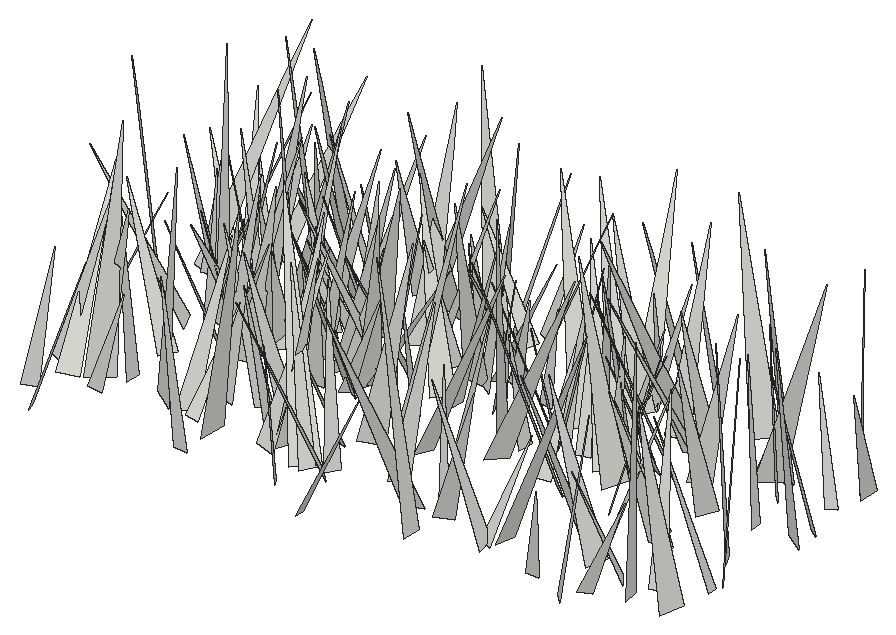
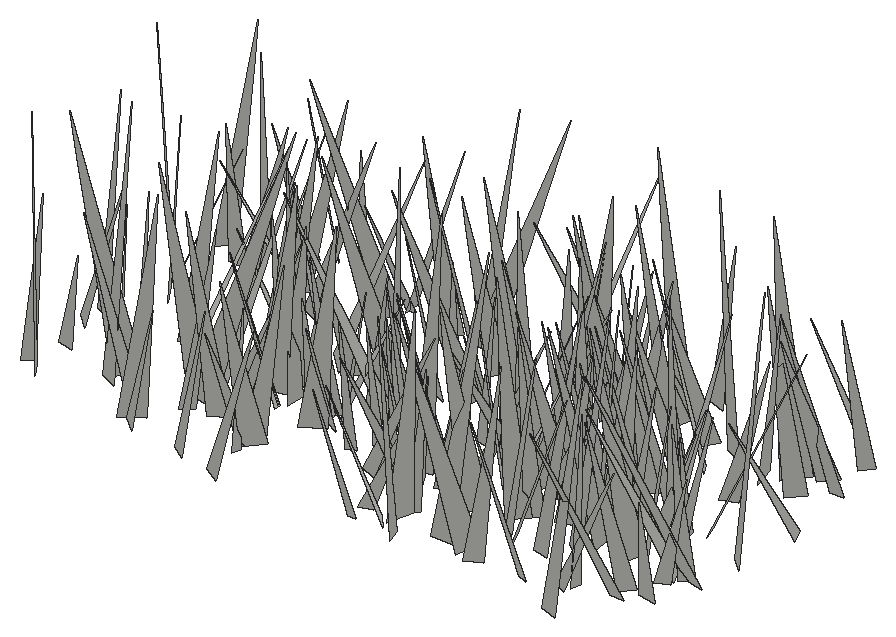
# SketchUp Ruby script. Lengths in inches.
U = 1.inch
M = Sketchup.active_model
def pt(a) = Geom::Point3d.new(a.map { |v| v * U })
def face(e, loops, mat)
  f = e.add_face(loops[0].map { |a| pt(a) })
  loops[1..].each { |l| e.add_face(l.map { |a| pt(a) }).erase! }
  f.material = f.back_material = mat if mat
  f
end
# faces: each face lists its corners as indices into pts; further lists are holes
def faces(e, pts, list, mat = nil) = list.each { |f| face(e, (f[0].is_a?(Array) ? f : [f]).map { |l| l.map { |i| pts[i] } }, mat) }
# xy, xz, yz: faces in a plane at the given z, y or x. An outline is a flat list of corners, or four numbers for a rectangle; further outlines are holes
def ring(l) = l.size == 4 ? [[l[0], l[1]], [l[2], l[1]], [l[2], l[3]], [l[0], l[3]]] : l.each_slice(2).to_a
def flat(e, list, mat, &to3) = list.each { |f| face(e, (f[0].is_a?(Array) ? f : [f]).map { |l| ring(l).map { |u, v| to3.(u, v) } }, mat) }
def xy(e, z, list, mat = nil) = flat(e, list, mat) { |x, y| [x, y, z] }
def xz(e, y, list, mat = nil) = flat(e, list, mat) { |x, z| [x, y, z] }
def yz(e, x, list, mat = nil) = flat(e, list, mat) { |y, z| [x, y, z] }
def lines(e, pts, list) = list.each { |a, b| e.add_line(pt(pts[a]), pt(pts[b])) }
# prism: a flat outline (further loops are holes) pulled along v
def prism(e, loops, v, mat = nil)
  f = face(e, loops, mat); d = Geom::Vector3d.new(v.map { |x| x * U })
  f.pushpull(f.normal.samedirection?(d) ? d.length : -d.length)
end
def box(e, o, s, mat = nil) = prism(e, [[o, [o[0] + s[0], o[1], o[2]], [o[0] + s[0], o[1] + s[1], o[2]], [o[0], o[1] + s[1], o[2]]]], [0, 0, s[2]], mat)
def at(x, y, z, deg = 0) = Geom::Transformation.translation(pt([x, y, z])) * Geom::Transformation.rotation(ORIGIN, Z_AXIS, deg.degrees)
def axes(o, x, y, z) = Geom::Transformation.new([*x, 0, *y, 0, *z, 0, *pt(o).to_a, 1])
def part(name) = M.definitions.add(name)
# library, detail: a bought-in or finely detailed component or shape, given as its bounding box
def library(name, o, s) = part(name).tap { |d| box(d.entities, o, s) }
def detail(e, o, s) = box(e.add_group.entities, o, s)
def put(e, d, t, mat = nil) = e.add_instance(d, t).tap { |i| i.material = mat if mat }
def group(e, t, mat = nil) = e.add_group.tap { |g| g.transformation = t; g.material = mat if mat }.entities
root = M.entities
c1 = part("fur_instance\#9")
p = [[0.8125,0,1.79],[0.67,-0.02,1.48],[0,-0.11,0],[0,0.11,0]]
faces(c1.entities,p,[[0,1,2,3]])
put(root,c1,axes([525.23,306.68,-21.66],[4.11341,0.99659,0.14821],[0.94897,-4.04143,0.83763],[-0.33855,0.78037,4.1487]))
put(root,c1,axes([506.24,306.79,-21.66],[4.19181,1.99584,0.5753],[1.88629,-4.2003,0.82769],[-0.86965,0.50967,4.56832]))
put(root,c1,axes([515.68,308.2,-21.66],[-1.40726,-4.75955,2.034],[-5.17479,1.24906,-0.65748],[-0.10975,2.13481,4.91949]))
put(root,c1,axes([539.56,309.3,-21.66],[0.99148,-3.49866,0.36174],[-3.47594,-0.91715,0.65665],[0.53788,0.52224,3.57665]))
put(root,c1,axes([523.57,310.96,-21.66],[-4.47092,-4.93614,0.16266],[-4.90041,4.46105,0.68268],[0.61475,-0.33851,6.62484]))
put(root,c1,axes([504.69,308.63,-21.66],[-2.17172,3.54056,2.13295],[3.72846,2.71807,-0.7156],[1.78427,-1.37037,4.09143]))
put(root,c1,axes([529.65,311.23,-21.66],[0.11863,-7.1905,0.64579],[-7.08435,-0.24031,-1.37429],[-1.39009,0.61104,7.05894]))
put(root,c1,axes([522,308.61,-21.66],[-3.20539,-1.99252,1.2784],[-2.28309,3.17085,-0.78241],[0.62603,1.36182,3.69222]))
put(root,c1,axes([543.06,309.57,-21.66],[3.00481,-2.76961,0.12717],[-2.71494,-2.90128,0.96303],[0.56213,0.79222,3.97142]))
put(root,c1,axes([542.36,308.125,-21.66],[3.86177,3.77021,1.4507],[3.73701,-4.09632,0.69796],[-1.5342,-0.48777,5.35169]))
put(root,c1,axes([535.49,310.27,-21.66],[-5.30182,-0.75056,0.88287],[-0.65483,5.35184,0.61739],[0.95603,-0.49663,5.31898]))
put(root,c1,axes([531.5,308.73,-21.66],[-7.85501,-1.13743,1.66782],[-1.3997,7.89692,-1.20666],[1.45472,1.45652,7.84468]))
put(root,c1,axes([548.03,311,-21.66],[-6.01027,1.97565,2.91231],[2.62602,6.35479,1.10849],[2.3428,-2.05464,6.22879]))
put(root,c1,axes([515.82,310.82,-21.66],[7.89082,-0.9052,1.78608],[-0.78265,-8.07818,-0.63641],[-1.84308,-0.44515,7.91703]))
put(root,c1,axes([531.8,311.22,-21.66],[3.60736,-4.41491,0.21347],[-4.38405,-3.53869,0.89879],[0.56311,0.73233,5.62998]))
put(root,c1,axes([507.74,310.5625,-21.66],[1.20072,-3.47995,0.99765],[-3.52529,-0.88496,1.15597],[0.82322,1.28603,3.49507]))
put(root,c1,axes([543.75,312.04,-21.66],[-3.41692,-2.65793,0.41527],[-2.50813,3.39027,1.06197],[0.9728,-0.5949,4.19669]))
put(root,c1,axes([535.33,310.45,-21.66],[0.85166,3.52496,0.51911],[3.494,-0.72175,-0.83136],[0.69768,-0.68839,3.5298]))
put(root,c1,axes([511.42,312.01,-21.66],[-3.32783,-6.52848,3.29816],[-6.89122,4.01297,0.99019],[2.45153,2.41834,7.26051]))
put(root,c1,axes([541.49,312.54,-21.66],[-5.54142,2.04017,2.02802],[2.50487,5.58649,1.22443],[1.41448,-1.90035,5.77671]))
put(root,c1,axes([545.33,310.76,-21.66],[-6.71268,-1.89599,2.76742],[-2.51748,6.93875,-1.3526],[2.21714,2.13833,6.8429]))
put(root,c1,axes([507.07,311.85,-21.66],[-5.12716,5.45276,3.67809],[5.84452,5.9162,-0.62364],[3.01704,-2.19425,7.45865]))
put(root,c1,axes([535.95,311.42,-21.66],[7.40622,-0.19557,0.80001],[-0.28757,-7.3972,0.85392],[-0.77173,0.87956,7.35943]))
put(root,c1,axes([522.49,310.92,-21.66],[-5.52094,1.92393,0.48296],[1.85996,5.5174,-0.71721],[0.68943,0.52184,5.80241]))
put(root,c1,axes([519.83,312.03,-21.66],[5.84499,-0.86217,1.83487],[-1.09003,-6.05756,0.62599],[-1.70936,0.91471,5.87498]))
put(root,c1,axes([505.89,313.43,-21.66],[3.45559,-4.90486,0.92565],[-4.98413,-3.32981,0.96246],[0.2699,1.30779,5.9222]))
put(root,c1,axes([513.93,311.37,-21.66],[-0.30009,3.62925,0.24074],[3.53668,0.34756,-0.831],[0.84929,-0.16496,3.54556]))
put(root,c1,axes([523.67,311.5625,-21.66],[-5.20641,1.3754,0.94823],[1.21962,5.25029,-0.91901],[1.14166,0.66356,5.30602]))
put(root,c1,axes([522.17,311.0625,-21.66],[-4.81407,6.51041,0.79127],[6.55623,4.75265,0.78417],[-0.16528,-1.10168,8.05889]))
put(root,c1,axes([504.21,311.87,-21.66],[1.48764,5.46016,1.29529],[5.56167,-1.25605,-1.09283],[0.74757,-1.52092,5.55267]))
put(root,c1,axes([519.22,311.18,-21.66],[1.31333,6.20143,0.89],[6.24264,-1.21867,-0.72041],[0.52849,-1.01577,6.2979]))
put(root,c1,axes([539.47,314.21,-21.66],[-1.836,-5.36618,0.72675],[-5.38286,1.72484,-0.86298],[-0.59066,0.96126,5.60554]))
put(root,c1,axes([513.17,311.84,-21.66],[-3.03856,4.16793,1.35783],[3.96538,3.31773,-1.3102],[1.86846,-0.26309,4.98878]))
put(root,c1,axes([517.71,313.45,-21.66],[-1.21907,-3.82959,1.50139],[-4.09681,0.98993,-0.80143],[-0.36895,1.66143,3.93822]))
put(root,c1,axes([505.54,310.92,-21.66],[-3.21539,5.33291,0.27404],[5.21793,3.20577,-1.16191],[1.13501,0.36996,6.11789]))
put(root,c1,axes([530.96,312.28,-21.66],[-3.9297,0.38452,0.60241],[0.18265,3.7953,-1.23109],[0.69093,1.18368,3.75164]))
put(root,c1,axes([527.22,312.97,-21.66],[4.47757,-3.00826,2.16701],[-3.51648,-4.52249,0.98776],[-1.1747,2.07164,5.30307]))
put(root,c1,axes([508.57,312.87,-21.66],[-5.92753,-0.80933,1.51712],[-1.07571,5.99367,-1.00549],[1.34146,1.2301,5.89742]))
put(root,c1,axes([522.33,314.2,-21.66],[-2.45002,-3.17903,0.27674],[-3.09062,2.27713,-1.20338],[-0.79426,0.94543,3.82893]))
put(root,c1,axes([546.05,312.3,-21.66],[-0.40963,5.6712,0.85204],[5.69515,0.30195,0.72827],[-0.67361,-0.89587,5.63914]))
put(root,c1,axes([519.03,313.05,-21.66],[-3.21117,5.73542,2.2751],[5.803,3.67883,-1.08356],[2.09673,-1.39782,6.48325]))
put(root,c1,axes([517.64,315.1875,-21.66],[-5.01187,1.13995,1.85475],[1.60842,5.07616,1.22637],[1.46717,-1.67079,4.99142]))
put(root,c1,axes([511.62,314.23,-21.66],[5.2265,3.38981,1.10604],[3.55749,-5.09026,-1.20993],[-0.2416,-1.62138,6.11091]))
put(root,c1,axes([513.7,314.26,-21.66],[1.63751,6.97927,2.94123],[7.53115,-1.18196,-1.38823],[0.80173,-3.15202,7.03309]))
put(root,c1,axes([548.45,314.0625,-21.66],[-4.94313,-1.68267,0.02369],[-1.64372,4.81198,-1.18726],[-0.36076,1.13137,5.08492]))
put(root,c1,axes([516.32,314.75,-21.66],[0.21554,-5.31829,2.18174],[-5.56977,-0.73327,-1.23719],[-1.42193,2.0661,5.17688]))
put(root,c1,axes([542.6875,316.59,-21.66],[1.51534,-5.37644,0.92666],[-5.31705,-1.67082,-0.99923],[-1.22223,0.60275,5.49581]))
put(root,c1,axes([548.05,315.53,-21.66],[-5.21121,-4.35385,3.58957],[-4.50193,6.15376,0.92827],[3.40202,1.4741,6.72689]))
put(root,c1,axes([541.59,312.71,-21.66],[4.07971,3.91858,0.07723],[3.79656,-3.97882,1.32677],[-0.97331,0.90496,5.499]))
put(root,c1,axes([523.4,315.33,-21.66],[4.4224,-5.22883,1.99199],[-5.58659,-4.26873,1.19762],[-0.31423,2.30295,6.7427]))
put(root,c1,axes([512.45,315.42,-21.66],[4.92372,-1.23429,0.65682],[-1.32256,-4.89156,0.72207],[-0.45359,0.86432,5.02445]))
put(root,c1,axes([536.63,317.3,-21.66],[3.04717,-2.22298,0.43436],[-2.028,-3.00193,-1.13631],[-1.00873,-0.67996,3.59662]))
put(root,c1,axes([542.6,317.14,-21.66],[-4.67386,-0.0885,1.27111],[0.2568,4.66814,1.26925],[1.24804,-1.29194,4.49909]))
put(root,c1,axes([510.14,318.6,-21.66],[-2.61623,-5.06997,0.16776],[-4.93297,2.58676,1.24576],[1.18261,-0.42604,5.56752]))
put(root,c1,axes([508.39,316.18,-21.66],[-3.73959,3.61146,1.09906],[3.77498,3.58144,1.07604],[0.00944,-1.53809,5.08619]))
put(root,c1,axes([543.7,316.25,-21.66],[-3.57996,-1.2077,0.30439],[-1.24532,3.48547,-0.8173],[0.0195,0.87192,3.68872]))
put(root,c1,axes([534.96,317.53,-21.66],[-5.01465,-5.39389,0.78065],[-5.43536,4.87162,-1.25473],[-0.40033,1.42249,7.25716]))
put(root,c1,axes([518.89,319.13,-21.66],[-2.89154,-5.8907,0.51675],[-5.81601,2.937,0.93617],[1.06836,0.04534,6.49499]))
put(root,c1,axes([526.29,316.31,-21.66],[6.61677,-1.08212,0.53072],[-1.15649,-6.53431,1.0953],[-0.3394,1.16883,6.6146]))
put(root,c1,axes([516.71,318.57,-21.66],[1.30695,-5.86281,0.96642],[-5.89292,-1.15208,0.98022],[0.76158,1.14664,5.9262]))
put(root,c1,axes([528.02,317.09,-21.66],[2.95558,3.83246,1.3061],[4.0436,-2.87668,-0.7093],[-0.20723,-1.47175,4.78749]))
put(root,c1,axes([512.33,318.21,-21.66],[4.00541,-4.88826,1.49079],[-5.10449,-3.91872,0.86522],[-0.24835,1.7057,6.26017]))
put(root,c1,axes([546.9,317.29,-21.66],[-5.34444,-2.84039,2.21318],[-3.30562,5.4408,-0.99979],[1.42788,1.96442,5.96919]))
put(root,c1,axes([506.96,319.625,-21.66],[-5.82237,-2.50943,0.01956],[-2.48564,5.77362,0.82736],[0.34528,-0.75212,6.28591]))
put(root,c1,axes([529.86,318.33,-21.66],[6.60673,-3.01857,0.44503],[-3.04917,-6.49303,1.22551],[0.11127,1.29906,7.15953]))
put(root,c1,axes([503.01,316.87,-21.66],[4.04294,1.47662,0.10602],[1.40514,-3.92456,1.07725],[-0.46609,0.97696,4.16717]))
put(root,c1,axes([512.49,319.57,-21.66],[1.67883,-4.20753,0.33675],[-4.18563,-1.61266,0.71764],[0.54516,0.57551,4.47289]))
put(root,c1,axes([519.27,320.28,-21.66],[6.44633,-3.37101,0.63256],[-3.2949,-6.46051,-0.8512],[-0.95262,-0.46602,7.22457]))
put(root,c1,axes([523.14,319.53,-21.66],[-1.38247,-3.90181,0.99129],[-3.91317,1.54858,0.63797],[0.94545,0.70412,4.09003]))
put(root,c1,axes([512.81,320.72,-21.66],[4.57924,-4.33247,0.58798],[-4.22206,-4.60304,-1.03525],[-1.13589,-0.35667,6.21836]))
put(root,c1,axes([518.7,318.98,-21.66],[3.23817,-2.36152,0.30304],[-2.37388,-3.16317,0.7165],[0.18248,0.75624,3.94324]))
put(root,c1,axes([515.875,319.8,-21.66],[3.30583,-2.31707,0.74955],[-2.21165,-3.38553,-0.71128],[-1.01942,-0.16893,3.97384]))
put(root,c1,axes([524.41,317.23,-21.66],[1.50713,3.43781,0.3216],[3.3001,-1.53741,0.96906],[-1.01552,0.10596,3.62641]))
put(root,c1,axes([523.75,317.8,-21.66],[-3.45696,-5.56122,4.74392],[-6.59951,4.63089,0.61955],[3.14299,3.60698,6.51874]))
put(root,c1,axes([542.74,320.71,-21.66],[4.44508,-4.04211,0.97735],[-3.87336,-4.54492,-1.18043],[-1.51359,-0.24009,5.89101]))
put(root,c1,axes([538.5,317.4,-21.66],[3.62249,2.81644,0.55831],[2.6251,-3.61284,1.19278],[-1.16313,0.61769,4.43081]))
put(root,c1,axes([533.35,318.03,-21.66],[-1.89071,3.52857,0.74513],[3.44423,2.01617,-0.80816],[1.06925,-0.25501,3.92077]))
put(root,c1,axes([536.8,320.03,-21.66],[-6.28621,2.90163,2.83322],[3.4688,6.55463,0.9835],[2.10096,-2.14018,6.85337]))
put(root,c1,axes([519.8125,321.31,-21.66],[-5.72076,-3.26575,0.35826],[-3.1922,5.6955,0.94426],[0.77675,-0.64548,6.51924]))
put(root,c1,axes([514.8,319.24,-21.66],[2.68991,-2.47286,1.2383],[-2.72716,-2.65872,0.6147],[-0.45937,1.30393,3.60178]))
put(root,c1,axes([528.72,320.23,-21.66],[6.72646,1.81373,2.96578],[2.30607,-7.16166,-0.85049],[-2.60144,-1.65881,6.91459]))
put(root,c1,axes([530.28,320.27,-21.66],[3.55115,-1.15094,1.45453],[-0.93925,-3.82501,-0.73353],[-1.59941,-0.30919,3.66022]))
put(root,c1,axes([520.47,320.61,-21.66],[1.50872,-3.69838,0.31644],[-3.67115,-1.43625,0.71715],[0.54852,0.55997,3.92937]))
put(root,c1,axes([510.64,318.49,-21.66],[5.6278,2.51424,1.57514],[2.22036,-5.80941,1.3399],[-1.96786,0.63554,6.01649]))
put(root,c1,axes([517.78,320.11,-21.66],[-0.77592,-4.15559,2.31409],[-4.39268,1.52537,1.26634],[1.82437,1.90534,4.03328]))
put(root,c1,axes([503.63,321.42,-21.66],[-5.15951,-5.90719,2.53837],[-5.9684,5.61072,0.92562],[2.3909,1.25844,7.78837]))
put(root,c1,axes([538.63,322.8125,-21.66],[-4.50054,-5.78959,0.45114],[-5.68851,4.51005,1.13049],[1.1678,-0.3432,7.24542]))
put(root,c1,axes([548.48,321.16,-21.66],[-3.10043,-5.65859,2.0595],[-5.81568,3.41455,0.62657],[1.56175,1.48157,6.42182]))
put(root,c1,axes([508.82,321.92,-21.66],[1.51991,-3.61395,0.26794],[-3.4425,-1.53065,-1.11749],[-1.13207,-0.1975,3.75792]))
put(root,c1,axes([509.875,320.1,-21.66],[-3.12705,-1.8127,0.50032],[-1.87769,2.95706,-1.02213],[-0.10232,1.13341,3.46693]))
put(root,c1,axes([521.29,321.94,-21.66],[-1.6318,-4.41068,0.10105],[-4.3461,1.58854,-0.8456],[-0.75876,0.38671,4.62621]))
put(root,c1,axes([535.83,321.03,-21.66],[0.28341,4.29415,2.46111],[4.89058,0.13603,-0.80051],[0.76092,-2.47364,4.22839]))
put(root,c1,axes([537.6875,320.58,-21.66],[-3.61019,-4.99925,2.09321],[-5.40705,3.49453,-0.97958],[0.37125,2.28107,6.08822]))
put(root,c1,axes([540.94,323.39,-21.66],[-5.31992,-4.92486,0.01845],[-4.88394,5.27914,0.91325],[0.63384,-0.65774,7.19179]))
put(root,c1,axes([512.74,320.28,-21.66],[-2.01026,5.06538,1.49078],[5.275,1.85579,0.80751],[-0.23431,-1.67916,5.38954]))
put(root,c1,axes([518.76,321.62,-21.66],[-2.91318,-3.12111,0.33199],[-3.12229,2.8354,-0.74159],[-0.32068,0.74655,4.20452]))
put(root,c1,axes([517.14,320.71,-21.66],[6.46627,-2.11143,1.67342],[-2.36842,-6.52888,0.91405],[-1.28416,1.40953,6.74057]))
put(root,c1,axes([515.45,320.88,-21.66],[5.24089,-0.83273,1.62957],[-1.05437,-5.41429,0.62423],[-1.49573,0.89885,5.2698]))
put(root,c1,axes([534.05,322.27,-21.66],[6.7511,0.38921,2.10678],[0.68602,-6.99103,-0.90679],[-2.02963,-1.06837,6.70124]))
put(root,c1,axes([519.35,320.49,-21.66],[4.38555,-0.36882,0.03632],[-0.36139,-4.16033,1.38975],[0.08213,1.3878,4.17584]))
put(root,c1,axes([531.47,321.92,-21.66],[5.91305,2.63208,1.30513],[2.84881,-5.85376,-1.10147],[-0.71801,-1.54954,6.37799]))
put(root,c1,axes([508.86,320.41,-21.66],[2.99088,7.34321,2.70362],[7.47912,-3.53374,1.32409],[-2.30112,-1.94104,7.81761]))
put(root,c1,axes([530.29,322.79,-21.66],[-2.2334,-3.12116,0.78897],[-3.02774,2.36275,0.77617],[1.09405,0.16724,3.75863]))
put(root,c1,axes([531.11,321.87,-21.66],[-3.78552,-3.06993,0.30173],[-3.01727,3.58565,-1.37288],[-0.64154,1.25071,4.67652]))
put(root,c1,axes([545.77,321.22,-21.66],[-4.75488,-0.89522,1.48594],[-1.16705,4.85843,-0.80746],[1.28353,1.10117,4.77057]))
put(root,c1,axes([537.71,322.61,-21.66],[-2.11494,-3.26023,0.3236],[-3.25153,2.04149,-0.68318],[-0.40176,0.64034,3.82562]))
put(root,c1,axes([507.64,320.73,-21.66],[-4.10668,0.43412,1.0008],[0.12519,4.05996,-1.24738],[1.0837,1.17608,3.93666]))
put(root,c1,axes([509.49,321.6,-21.66],[3.29943,5.39851,1.49465],[5.593,-3.07886,-1.22601],[0.31023,-1.9081,6.20701]))
put(root,c1,axes([523.73,324.16,-21.66],[0.64901,-7.30772,0.94418],[-7.33385,-0.54888,0.79295],[0.71332,1.00569,7.2935]))
put(root,c1,axes([531.41,322.14,-21.66],[-0.36242,4.3186,2.109],[4.6668,0.82166,-0.88056],[1.14855,-1.97588,4.24338]))
put(root,c1,axes([514.19,323.77,-21.66],[-2.66612,-3.28273,0.28859],[-3.19335,2.6653,0.81637],[0.81369,-0.29607,4.14946]))
put(root,c1,axes([514.14,320.26,-21.66],[2.11808,6.39246,0.96016],[6.39192,-2.22182,0.69185],[-0.96378,-0.68681,6.6986]))
put(root,c1,axes([519.23,322.48,-21.66],[4.62058,2.87983,1.50344],[3.15499,-4.60106,-0.88304],[-0.77446,-1.56215,5.37246]))
put(root,c1,axes([535.46,320.94,-21.66],[-3.34888,5.66427,0.75226],[5.70524,3.26636,0.80369],[-0.31635,-1.05439,6.53093]))
put(root,c1,axes([548.75,322.59,-21.66],[-3.27995,-3.84872,1.10692],[-4.00472,3.15616,-0.89264],[0.01123,1.42196,4.97734]))
put(root,c1,axes([513.25,321.55,-21.66],[-6.49961,-2.89491,2.26898],[-3.37847,6.5202,-1.35892],[1.4542,2.20912,6.98418]))
put(root,c1,axes([528.58,320.72,-21.66],[7.17048,3.0592,0.30714],[3.02615,-7.16002,0.66735],[-0.54355,0.49421,7.76718]))
put(root,c1,axes([513.13,322.95,-21.66],[3.69206,0.52175,1.19179],[0.74035,-3.79133,-0.63373],[-1.0698,-0.8231,3.6745]))
put(root,c1,axes([526.38,323.17,-21.66],[-1.07299,-3.39329,1.1863],[-3.30809,1.41653,1.05972],[1.4065,0.74301,3.39746]))
put(root,c1,axes([518.68,322.47,-21.66],[-4.50374,-2.5863,0.2222],[-2.55985,4.35118,-1.23954],[-0.43072,1.18335,5.04343]))
put(root,c1,axes([510.92,321.62,-21.66],[-5.72971,0.10944,0.75393],[-0.02545,5.68949,-1.01935],[0.7614,1.01378,5.63937]))
put(root,c1,axes([524.35,321.6875,-21.66],[5.06172,0.87175,1.3003],[0.68802,-5.19178,0.80241],[-1.40619,0.59773,5.07318]))
put(root,c1,axes([538.15,325.53,-21.66],[0.33917,-8.30019,0.61155],[-8.21231,-0.43312,-1.32383],[-1.35096,0.54903,8.20095]))
put(root,c1,axes([540.37,323.01,-21.66],[-2.5167,4.57974,3.46384],[4.9953,3.61127,-1.14527],[2.83182,-2.30014,5.09864]))
put(root,c1,axes([536.55,323.59,-21.66],[-2.94659,-4.28728,0.79485],[-4.35538,2.84813,-0.78348],[-0.2081,1.09651,5.14289]))
put(root,c1,axes([534.41,323.41,-21.66],[4.26627,1.55205,0.05399],[1.49304,-4.05567,-1.39111],[0.42732,-1.32496,4.32143]))
put(root,c1,axes([533.4,321.49,-21.66],[-0.37252,4.33667,0.3989],[4.3129,0.31185,0.63743],[-0.60398,-0.44793,4.30572]))
put(root,c1,axes([506.41,323.2,-21.66],[-1.858,-4.3991,1.45242],[-4.62148,1.65138,-0.9103],[-0.32175,1.68364,4.68782]))
put(root,c1,axes([523.21,321.86,-21.66],[-3.60307,5.2202,0.86904],[5.28801,3.51043,0.83765],[-0.20649,-1.18922,6.28736]))
put(root,c1,axes([515.35,324,-21.66],[0.6602,-3.48398,0.63366],[-3.31771,-0.83389,-1.12823],[-1.23791,0.37685,3.36171]))
put(root,c1,axes([513.87,323.69,-21.66],[2.18387,-4.44969,1.85832],[-4.59717,-2.53702,-0.67228],[-1.45572,1.33648,4.91091]))
put(root,c1,axes([516.2,324.92,-21.66],[4.17782,-5.39394,0.17375],[-5.37681,-4.14138,0.71959],[0.46328,0.57738,6.78461]))
put(root,c1,axes([526.45,322.29,-21.66],[2.93854,2.24557,1.05284],[2.03507,-3.11619,0.96641],[-1.41759,0.18132,3.56983]))
put(root,c1,axes([514.12,322.63,-21.66],[6.01682,-1.89651,1.60783],[-2.22,-5.99358,1.23799],[-1.11958,1.69241,6.18597]))
put(root,c1,axes([534.85,323.05,-21.66],[2.48119,3.58815,0.88423],[3.68479,-2.32113,-0.92071],[0.2811,-1.24521,4.2642]))
put(root,c1,axes([535.73,322.22,-21.66],[-3.99948,7.12267,1.32626],[7.23474,3.8453,1.16596],[-0.38726,-1.72292,8.0851]))
put(root,c1,axes([521.6,324.85,-21.66],[3.25434,-3.10316,1.28908],[-2.93626,-3.49873,-1.00964],[-1.63392,0.10675,4.38189]))
put(root,c1,axes([515.64,324.26,-21.66],[2.0151,-5.02328,1.60572],[-5.27188,-1.87389,0.75376],[0.13771,1.76848,5.35965]))
put(root,c1,axes([524.39,324.04,-21.66],[2.41252,4.65389,1.89869],[5.02303,-2.30836,-0.72433],[-0.1815,-2.02404,5.19175]))
put(root,c1,axes([528.28,324.63,-21.66],[0.50859,-3.54434,0.97529],[-3.61365,-0.30136,0.78924],[0.67458,1.05784,3.49258]))
put(root,c1,axes([504.6,324.6,-21.66],[1.60896,-4.17155,1.4473],[-4.41412,-1.4813,0.63763],[0.1098,1.57772,4.42538]))
put(root,c1,axes([525.55,325.3,-21.66],[0.50493,-3.90237,0.56248],[-3.75126,-0.30094,1.27958],[1.21364,0.69337,3.72104]))
put(root,c1,axes([506.88,325.58,-21.66],[-3.29784,-3.61715,1.25797],[-3.53735,3.51322,0.8285],[1.46745,0.33986,4.82422]))
put(root,c1,axes([530.68,323.25,-21.66],[1.32341,3.79294,0.4756],[3.74321,-1.38791,0.65276],[-0.77522,-0.22654,3.9638]))
put(root,c1,axes([525.92,326,-21.66],[-1.33885,-4.31341,0.19295],[-4.24788,1.27969,-0.86785],[-0.77346,0.43835,4.43226]))
put(root,c1,axes([544.67,324.43,-21.66],[-3.59286,-3.26733,2.03566],[-3.70516,3.69058,-0.61592],[1.04455,1.85261,4.81713]))
put(root,c1,axes([531.43,323.97,-21.66],[-4.74257,5.72398,1.5327],[5.90767,4.72004,0.65254],[0.46105,-1.60076,7.40474]))
put(root,c1,axes([510.79,324.16,-21.66],[6.83211,0.09479,1.62922],[-0.11306,-6.96812,0.87954],[-1.62805,0.88169,6.77592]))
put(root,c1,axes([508.46,324.47,-21.66],[6.64236,-2.17739,2.19825],[-2.53423,-6.81539,0.90685],[-1.77512,1.5823,6.93106]))
put(root,c1,axes([512.82,327.25,-21.66],[-2.64137,-6.46023,1.04071],[-6.35863,2.79897,1.23619],[1.54452,0.47506,6.86901]))
put(root,c1,axes([543.1875,325.55,-21.66],[6.11915,-4.70581,1.11272],[-4.83462,-5.98952,1.25659],[-0.09634,1.67568,7.61641]))
put(root,c1,axes([515.76,326.32,-21.66],[-2.72161,-4.19987,1.18368],[-4.18397,2.90781,0.69726],[1.23872,0.59401,4.95579]))
put(root,c1,axes([538.14,326.66,-21.66],[-4.48343,0.78051,2.64752],[1.64873,4.80743,1.37477],[2.21365,-1.99978,4.33824]))
put(root,c1,axes([543.55,326.83,-21.66],[-3.953,-6.85404,2.35159],[-6.87911,4.39144,1.23577],[2.27722,1.36799,7.81517]))
put(root,c1,axes([522.89,324.91,-21.66],[-3.3024,-1.44134,1.34219],[-1.74105,3.36144,-0.674],[0.92071,1.18661,3.53964]))
put(root,c1,axes([519.98,325.39,-21.66],[4.42305,4.26534,0.99754],[4.37397,-4.22348,-1.33498],[0.23791,-1.64944,5.99786]))
put(root,c1,axes([511.37,326.02,-21.66],[-4.43723,-6.45792,2.6794],[-6.95056,4.4181,-0.86196],[0.75734,2.71083,7.78786]))
put(root,c1,axes([505.51,325.64,-21.66],[-2.80157,3.07223,0.58027],[3.12461,2.72376,0.66487],[-0.11008,-0.87559,4.10431]))
put(root,c1,axes([524.36,325.09,-21.66],[4.0884,0.15219,0.34801],[0.0557,-3.96154,1.07814],[-0.37573,1.0688,3.94662]))
put(root,c1,axes([548.45,327.8,-21.66],[4.29129,-1.7599,0.57931],[-1.53313,-4.1935,-1.38278],[-1.04037,-1.07949,4.42723]))
put(root,c1,axes([547.8,325.33,-21.66],[-0.43735,3.78387,0.74816],[3.7266,0.2203,1.06426],[-0.99494,-0.83814,3.65736]))
put(root,c1,axes([505.51,324.39,-21.66],[5.65943,2.62486,0.30549],[2.50558,-5.55953,1.3513],[-0.8398,1.10185,6.0904]))
put(root,c1,axes([541.65,327.13,-21.66],[5.27208,0.02621,0.0042],[0.02652,-5.23568,-0.61848],[-0.0011,-0.61849,5.23574]))
put(root,c1,axes([518.01,329.4,-21.66],[-1.4202,-8.16889,0.91065],[-8.13373,1.52988,1.03868],[1.18423,0.71114,8.22611]))
put(root,c1,axes([514.89,326.96,-21.66],[-5.1041,-1.8904,0.52095],[-1.9461,5.06157,-0.70004],[0.24022,0.83889,5.39772]))
put(root,c1,axes([521.18,327.95,-21.66],[3.43553,-2.13589,0.95207],[-2.02418,-3.56342,-0.68999],[-1.17096,-0.10667,3.98608]))
put(root,c1,axes([536.22,326.25,-21.66],[-1.99924,6.11191,2.2816],[6.3463,2.375,-0.80119],[1.51181,-1.88733,6.38047]))
put(root,c1,axes([518.68,325.6,-21.66],[5.55139,-3.03279,3.66915],[-4.09539,-5.91606,1.30628],[-2.42657,3.04644,6.18946]))
put(root,c1,axes([533.04,327.16,-21.66],[-4.86777,3.35697,1.6535],[3.6105,4.92638,0.62739],[0.98366,-1.46972,5.8797]))
put(root,c1,axes([504.14,324.65,-21.66],[2.50136,7.65725,0.1478],[7.63522,-2.48107,-0.67805],[0.59891,-0.35058,8.02686]))
put(root,c1,axes([506.51,327.51,-21.66],[2.49544,-4.2024,1.5625],[-4.46283,-2.15679,1.32672],[0.42981,2.0042,4.70396]))
put(root,c1,axes([547.34,328.48,-21.66],[6.08028,3.66314,2.96745],[4.34842,-6.22849,-1.22118],[-1.82087,-2.64225,6.99265]))
put(root,c1,axes([508.99,328.89,-21.66],[4.7247,0.27251,1.48983],[0.66278,-4.76043,-1.23114],[-1.36183,-1.37139,4.56961]))
put(root,c1,axes([533.07,328.67,-21.66],[3.93197,-0.07434,1.3447],[0.21137,-4.06439,-0.84276],[-1.33006,-0.86567,3.84131]))
put(root,c1,axes([515.14,330.24,-21.66],[4.0127,-3.86264,0.72099],[-3.71726,-4.06564,-1.09277],[-1.27351,-0.30356,5.46147]))
put(root,c1,axes([509.64,329.5,-21.66],[-1.12963,-3.6746,0.26296],[-3.62855,1.06225,-0.74377],[-0.63679,0.46567,3.77168]))
put(root,c1,axes([533.15,327.78,-21.66],[3.71678,-0.58843,1.31141],[-0.99782,-3.67326,1.17982],[-1.0346,1.42876,3.57333]))
put(root,c1,axes([523.51,329.24,-21.66],[-3.19624,2.75407,0.40141],[2.73336,2.9911,1.24258],[-0.52417,-1.19599,4.03198]))
put(root,c1,axes([505.07,327.55,-21.66],[-0.56854,4.75375,0.07359],[4.64609,0.5398,1.02436],[-1.0087,-0.19303,4.67676]))
put(root,c1,axes([539.93,329.27,-21.66],[-5.03128,5.10175,2.45438],[5.52933,5.13327,0.66454],[1.21582,-2.23324,7.13442]))
put(root,c1,axes([516.28,329.3,-21.66],[6.91635,-1.96319,0.7746],[-2.05636,-6.86586,0.95992],[-0.47486,1.1384,7.12521]))
put(root,c1,axes([532.75,327.55,-21.66],[-3.90742,5.66938,0.63215],[5.60395,3.95813,-0.85923],[1.06639,-0.02677,6.83166]))
put(root,c1,axes([521.38,328.88,-21.66],[-7.28379,2.71503,1.56111],[2.64145,7.44897,-0.63058],[1.68261,0.05921,7.74773]))
put(root,c1,axes([520.37,330.74,-21.66],[5.81902,2.09502,1.94943],[2.48849,-5.88572,-1.1028],[-1.4131,-1.7377,6.08555]))
put(root,c1,axes([506.48,328.44,-21.66],[1.55452,5.85258,0.28483],[5.77094,-1.47817,-1.12324],[1.01494,-0.55917,5.95042]))
put(root,c1,axes([539.57,329.98,-21.66],[1.87721,3.55983,2.07479],[3.45548,-2.60202,1.33802],[-2.2443,-1.02868,3.79553]))
put(root,c1,axes([511.88,330,-21.66],[2.7927,4.03544,0.85961],[4.11922,-2.66751,-0.85986],[0.23622,-1.19268,4.83163]))
put(root,c1,axes([508.38,332.08,-21.66],[-2.6676,-6.3456,1.58153],[-6.4273,2.85927,0.63121],[1.20736,1.20081,6.85451]))
put(root,c1,axes([535.49,330.75,-21.66],[-2.59622,-3.87524,1.56211],[-4.17566,2.47102,-0.8099],[0.14666,1.75346,4.59368]))
put(root,c1,axes([523.5,330.5,-21.66],[1.6531,3.56586,0.9383],[3.65871,-1.45863,-0.90264],[0.45784,-1.21883,3.82535]))
put(root,c1,axes([532.53,331.58,-21.66],[-2.18314,-4.32344,1.23175],[-4.48368,1.99494,-0.94459],[-0.32548,1.51774,4.75036]))
put(root,c1,axes([521.85,329.84,-21.66],[3.70568,3.40586,0.49894],[3.35111,-3.73706,0.62078],[-0.78668,0.12425,4.99466]))
